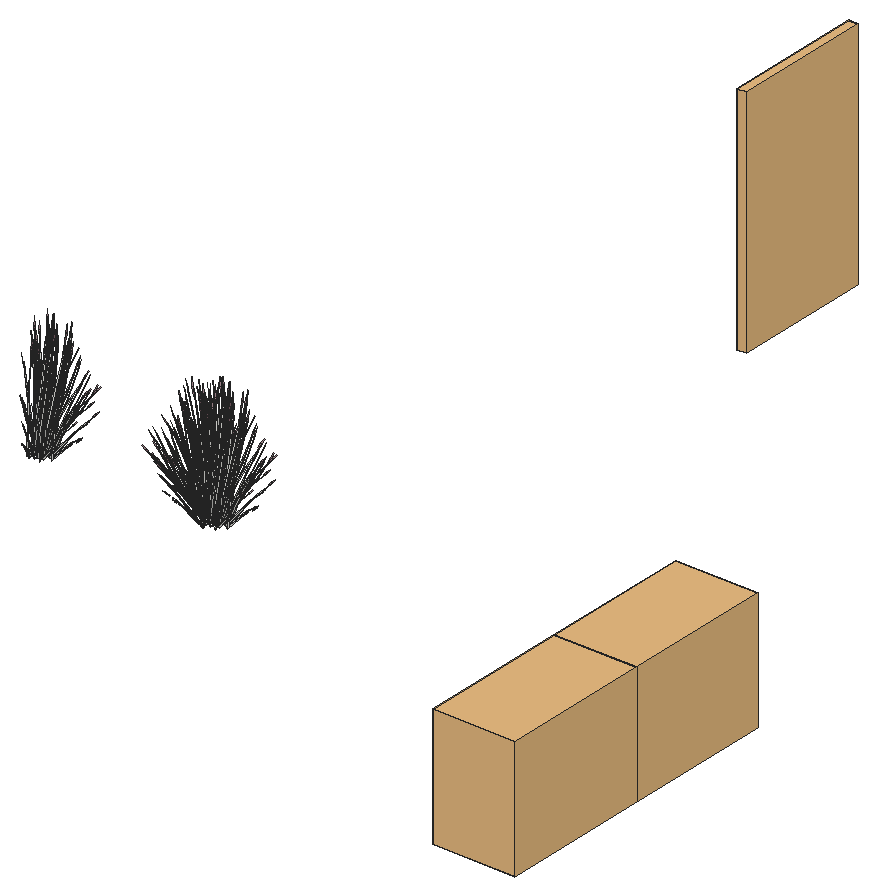
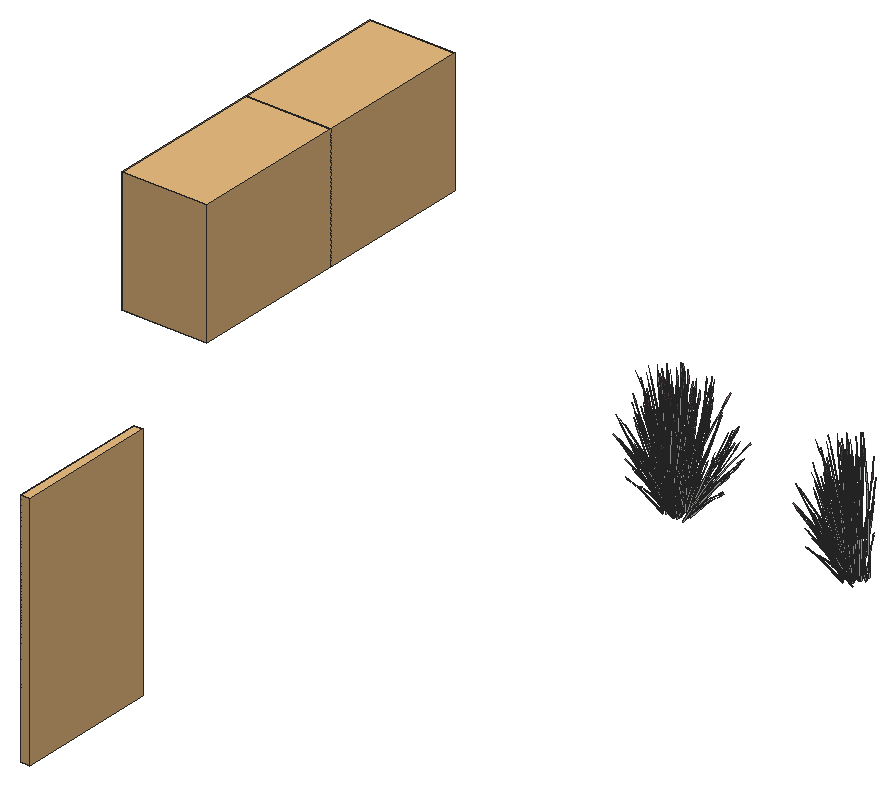
# SketchUp Ruby script. Lengths in millimetres.
U = 1.mm
M = Sketchup.active_model
def pt(a) = Geom::Point3d.new(a.map { |v| v * U })
def face(e, loops, mat)
  f = e.add_face(loops[0].map { |a| pt(a) })
  loops[1..].each { |l| e.add_face(l.map { |a| pt(a) }).erase! }
  f.material = f.back_material = mat if mat
  f
end
# faces: each face lists its corners as indices into pts; further lists are holes
def faces(e, pts, list, mat = nil) = list.each { |f| face(e, (f[0].is_a?(Array) ? f : [f]).map { |l| l.map { |i| pts[i] } }, mat) }
# xy, xz, yz: faces in a plane at the given z, y or x. An outline is a flat list of corners, or four numbers for a rectangle; further outlines are holes
def ring(l) = l.size == 4 ? [[l[0], l[1]], [l[2], l[1]], [l[2], l[3]], [l[0], l[3]]] : l.each_slice(2).to_a
def flat(e, list, mat, &to3) = list.each { |f| face(e, (f[0].is_a?(Array) ? f : [f]).map { |l| ring(l).map { |u, v| to3.(u, v) } }, mat) }
def xy(e, z, list, mat = nil) = flat(e, list, mat) { |x, y| [x, y, z] }
def xz(e, y, list, mat = nil) = flat(e, list, mat) { |x, z| [x, y, z] }
def yz(e, x, list, mat = nil) = flat(e, list, mat) { |y, z| [x, y, z] }
def lines(e, pts, list) = list.each { |a, b| e.add_line(pt(pts[a]), pt(pts[b])) }
# prism: a flat outline (further loops are holes) pulled along v
def prism(e, loops, v, mat = nil)
  f = face(e, loops, mat); d = Geom::Vector3d.new(v.map { |x| x * U })
  f.pushpull(f.normal.samedirection?(d) ? d.length : -d.length)
end
def box(e, o, s, mat = nil) = prism(e, [[o, [o[0] + s[0], o[1], o[2]], [o[0] + s[0], o[1] + s[1], o[2]], [o[0], o[1] + s[1], o[2]]]], [0, 0, s[2]], mat)
def at(x, y, z, deg = 0) = Geom::Transformation.translation(pt([x, y, z])) * Geom::Transformation.rotation(ORIGIN, Z_AXIS, deg.degrees)
def axes(o, x, y, z) = Geom::Transformation.new([*x, 0, *y, 0, *z, 0, *pt(o).to_a, 1])
def part(name) = M.definitions.add(name)
# library, detail: a bought-in or finely detailed component or shape, given as its bounding box
def library(name, o, s) = part(name).tap { |d| box(d.entities, o, s) }
def detail(e, o, s) = box(e.add_group.entities, o, s)
def put(e, d, t, mat = nil) = e.add_instance(d, t).tap { |i| i.material = mat if mat }
def group(e, t, mat = nil) = e.add_group.tap { |g| g.transformation = t; g.material = mat if mat }.entities
root = M.entities
M.materials.add("LightPink_Translucent").color = [144, 107, 117]
M.materials["LightPink_Translucent"].alpha = 0.8
c1 = part("blade")
p = [[54.7,5.3,558.8],[0,4.4,0],[2.3,11.5,0],[55.5,7.8,558.8],[58.2,7.8,558.8],[9.8,11.5,0],
  [62.9,5.7,838.2],[63,6,838.2],[63.4,6,838.2]]
faces(c1.entities,p,[[0,1,2,3],[4,5,2,3],[6,0,3,7],[7,3,4,8]])
c2 = part("seeds")
p = [[7.6,-2.7,35.1],[-0.2,-0.6,40.4],[-0.2,-0.8,0.9],[3.5,-1.8,-1.7],[7.5,-0.8,76.3],[3.7,0.2,78.9]]
faces(c2.entities,p,[[0,1,2,3],[1,0,4,5]],"LightPink_Translucent")
c3 = part("blade with seeds")
put(c3.entities,c1,at(0,0,0))
put(c3.entities,c2,axes([60.9,6.5,787.2],[1.5799,-0.05474,1.17369],[-0.12525,1.92788,0.29478],[-0.07173,-0.02425,1.56792]))
c4 = library("porta+4",[5.1,-137.5,33.9],[1182.3,119.8,2113.3])
c5 = library("Ornamental gate leaf",[0,0,0],[4100,1077.8,7119.6])
c6 = part("cong")
put(c6.entities,c5,axes([6217.3,5957.9,0],[-1,0,0],[0,1,0],[0,0,1]))
put(c6.entities,c5,at(6217.3,5957.9,0))
put(root,c3,axes([10117.4,4303.7,60],[0.53281,1.15808,0.45755],[-1.52239,0.4027,0.17955],[0.01861,-0.2128,1.58856]))
put(root,c3,axes([10111.2,4299.9,56.2],[0.59459,-0.93321,-0.44739],[1.23546,0.44912,0.21531],[0,-0.21512,1.43643]))
put(root,c3,axes([10149.9,4376.4,56],[-0.39985,-0.89288,0],[1.1418,-0.31268,0],[0,0,1.54371]))
put(root,c3,axes([10113,4424.2,37.9],[0.19833,-0.05635,1.76342],[1.19302,0.31018,-0.26939],[0.03489,0.3496,0.30037]))
put(root,c3,axes([10119.7,4432.2,115],[-0.36946,0.79643,-0.35414],[-1.07787,-0.23229,0.4572],[0.09883,0.32066,0.87481]))
put(root,c3,axes([10190.9,4331.6,56.2],[-0.59459,0.93321,-0.44739],[-1.23546,-0.44912,0.21531],[0,0.21512,1.43643]))
put(root,c3,axes([10250.6,4317.2,62.8],[-0.96285,-0.75439,0.17642],[0.97031,-0.7317,0.35086],[-0.10634,0.15406,1.60407]))
put(root,c3,axes([10166.1,4306.1,56],[0,-1.19833,0],[1.53239,0,0],[0,0,1.79456]))
put(root,c3,axes([10129.9,4311.7,61.8],[1.3808,0.50196,0.24065],[-0.66454,1.04299,0.50002],[0,-0.24043,1.60543]))
put(root,c3,axes([10185.7,4318.3,58.2],[0,1.19774,-0.05637],[-1.53239,0,0],[0,0.03764,1.79368]))
put(root,c3,axes([10118.6,4293.9,69],[-1.33077,0.06393,0.44739],[-0.12035,-1.06125,-0.21531],[0.23824,-0.10756,1.43643]))
put(root,c3,axes([10102.8,4247.7,62.8],[-0.35402,1.02926,0.17642],[-1.29548,-0.29127,0.35086],[0.22379,-0.00501,1.60407]))
put(root,c3,axes([10167.1,4377.2,58.2],[0.53281,1.18979,-0.06012],[-1.52239,0.41691,0],[0.01861,0.04155,1.72173]))
put(root,c3,axes([10086.7,4215.4,60.3],[-0.7662,-1.03778,0],[1.28187,-0.57875,-0.51607],[0.29196,-0.13181,1.63711]))
put(root,c3,axes([10122.5,4414.1,126.5],[0.5849,0.8421,-0.71045],[-1.20401,0.4693,0.08574],[0.13677,0.40688,1.00501]))
put(root,c3,axes([10278.8,4337.5,55.9],[-1.53164,-0.00828,-0.04976],[0,-1.1575,0.49943],[-0.04813,0.2635,1.58352]))
put(root,c3,axes([10202.4,4249.1,62.8],[-1.31687,0.27488,0.17642],[-0.32517,-1.02297,0.35086],[0.11745,0.14905,1.60407]))
put(root,c3,axes([10168.2,4151.7,70.2],[0.15721,0.60392,1.1486],[-0.87211,-0.33448,0.84392],[0.09385,-0.30923,0.25299]))
put(root,c3,axes([10147.7,4287,60],[-1.01611,0.93987,0.45755],[-1.20717,-0.82966,0.17955],[0.24496,-0.0938,1.58856]))
put(root,c3,axes([10191.7,4324.6,56.2],[0.85545,0.66896,0],[-0.85545,0.66896,0],[0,0,1.69266]))
put(root,c3,axes([10191.4,4304.7,69],[0.59459,-0.93321,0.44739],[1.23546,0.44912,-0.21531],[0,0.21512,1.43643]))
put(root,c3,axes([10178.3,4387.1,56],[1.23546,0.46496,0],[-0.59459,0.96613,0],[0,0,1.74954]))
put(root,c3,axes([10133.6,4418.4,118.9],[1.20468,0.25962,-0.51099],[-0.41292,0.89013,-0.3958],[0.11046,0.35838,0.97773]))
put(root,c3,axes([10181.3,4299.1,60.5],[-1.54892,-0.2182,0.49198],[0.31522,-1.23236,0.19306],[0.22636,0.119,1.70813]))
put(root,c3,axes([10270.7,4341.8,51.5],[-0.85545,0.64616,-0.30978],[-0.85545,-0.64616,0.30978],[0,0.20813,1.38974]))
put(root,c3,axes([10208.6,4338.8,53.2],[0.44936,0.94823,-0.69212],[-1.29441,0.3415,-0.18165],[0.04967,0.32109,1.52773]))
put(root,c3,axes([10192.5,4313,56],[1.37109,0,0],[0,1.07219,0],[0,0,1.78407]))
put(root,c3,axes([10159,4282.9,69],[-0.73619,-0.86927,0.44739],[1.11511,-0.61213,-0.21531],[0.23824,0.10756,1.43643]))
put(root,c3,axes([10125,4288.2,67.7],[-0.1428,-1.18174,-0.29095],[1.48733,-0.07145,-0.50002],[0.26191,-0.15741,1.59708]))
put(root,c3,axes([10204.6,4310.2,66.5],[1.1418,-0.30203,0.1448],[0.39985,0.86246,-0.41347],[0,0.18981,1.26744]))
put(root,c3,axes([10215.4,4225.5,118.9],[-0.87728,-0.69587,-0.51099],[0.92674,-0.60943,-0.3958],[0.13348,-0.35356,0.97773]))
put(root,c3,axes([10194.6,4311.9,67.7],[1.38012,0.49416,-0.29095],[-0.66454,1.04299,-0.50002],[0.04337,0.25608,1.59708]))
put(root,c3,axes([10120,4221.7,51.5],[1.14332,0.25625,-0.30978],[-0.28787,0.90242,0.30978],[0.23049,-0.10406,1.38974]))
put(root,c3,axes([10200.8,4194.1,65.8],[-0.34835,0.20963,1.43002],[-1.04325,-0.36691,-0.30754],[0.19338,-0.4563,0.61141]))
put(root,c3,axes([10270.7,4318,63],[0,-1.03566,0.49651],[1.37109,0,0],[0,0.23588,1.57504]))
put(root,c3,axes([10285.7,4342.4,51.2],[0,1.03566,-0.49651],[-1.37109,0,0],[0,0.23588,1.57504]))
put(root,c3,axes([10113.2,4211.3,51.2],[1.14694,-0.51783,-0.49651],[0.68554,0.92854,0],[0.26122,-0.11794,1.57504]))
put(root,c3,axes([10151,4371.7,98.5],[-0.28013,-0.33252,1.71376],[1.29445,-0.27994,0.13857],[0.29256,0.52202,0.73262]))
put(root,c3,axes([10171.6,4276.7,66.5],[0.23642,-0.92427,0.1448],[1.15506,0.16044,-0.41347],[0.21021,0.09491,1.26744]))
put(root,c3,axes([10213.3,4235.8,63],[-1.14694,-0.51783,0.49651],[0.68554,-0.92854,0],[0.26122,0.11794,1.57504]))
put(root,c3,axes([10222.3,4233.5,126.5],[0.03189,-0.95798,-0.71045],[1.34277,0.06434,0.08574],[0.14171,-0.40585,1.00501]))
put(root,c3,axes([10187.9,4373.2,55.5],[1.2866,-0.3514,-0.19198],[0.45209,1.01223,0.00008],[0.14202,-0.03884,1.73897]))
put(root,c3,axes([10188.5,4296.7,56.2],[0.73619,0.86927,-0.44739],[-1.11511,0.61213,0.21531],[0.23824,0.10756,1.43643]))
put(root,c3,axes([10236.4,4218.9,115],[0.82919,-0.54528,-0.35414],[0.78493,0.62262,0.4572],[0.11943,-0.31634,0.87481]))
put(root,c3,axes([10241.4,4397,70.2],[-0.69001,-0.29779,1.1486],[0.89096,-0.30257,0.84392],[0.24031,0.2563,0.25299]))
put(root,c3,axes([10179,4388.9,65.8],[0.02163,-0.34331,1.43002],[1.03345,-0.38348,-0.30754],[0.31903,0.4109,0.61141]))
put(root,c3,axes([10147.7,4265.3,52.3],[0.82544,-0.77843,-0.62353],[1.0254,0.70586,-0.16365],[0.33076,-0.19418,1.37633]))
put(root,c3,axes([10239.7,4247.7,51.5],[0.28787,0.90242,-0.30978],[-1.14332,0.25625,0.30978],[0.23049,0.10406,1.38974]))
put(root,c3,axes([10294.4,4322.4,60.4],[1.53239,0,0],[0,1.1575,-0.51607],[0,0.26363,1.63711]))
put(root,c3,axes([10168.6,4284.3,67.7],[1.23732,-0.68758,-0.29095],[0.8228,0.97154,-0.50002],[0.30528,0.09867,1.59708]))
put(root,c3,axes([10244.2,4431.4,67.7],[-0.78586,-0.03248,1.0506],[0.51898,-0.68985,0.58006],[0.31045,0.24509,0.8241]))
put(root,c3,axes([10184,4221.2,98.5],[-0.22818,0.35597,1.71376],[-0.95725,-0.73667,0.13857],[0.43183,-0.45914,0.73262]))
put(root,c3,axes([10089.2,4268.8,40.5],[-1.20625,0.41464,1.28929],[-0.38394,-1.1897,0.50096],[0.74071,0.01979,1.46642]))
put(root,c3,axes([10201.8,4407.4,118.9],[1.20928,-0.24619,-0.51099],[0.21154,0.93233,-0.3958],[0.32481,0.26718,0.97773]))
put(root,c3,axes([10230.1,4222,60.4],[0.7662,-1.03778,0],[1.28187,0.57875,-0.51607],[0.29196,0.13181,1.63711]))
put(root,c3,axes([10262.7,4210.5,37.9],[-0.18342,-0.08159,1.76342],[-0.47115,-0.9115,-0.26939],[0.31784,-0.24736,0.30037]))
put(root,c3,axes([10247.8,4237.9,51.2],[1.14694,0.51783,-0.49651],[-0.68554,0.92854,0],[0.26122,0.11794,1.57504]))
put(root,c3,axes([10246.4,4425,37.9],[0.08928,-0.14952,1.76342],[1.12407,-0.44035,-0.26939],[0.34078,0.22791,0.30037]))
put(root,c3,axes([10261.7,4266.1,118.9],[-0.31482,-0.94565,-0.51099],[1.19224,-0.16542,-0.3958],[0.34166,-0.254,0.97773]))
put(root,c3,axes([10315,4390.1,99.8],[-0.23455,-0.87059,-0.03492],[1.10861,-0.20015,-0.15832],[0.23151,0.05519,0.52218]))
put(root,c3,axes([10205.3,4288.3,52.3],[1.27479,0.1698,-0.62353],[-0.26901,1.04736,-0.16365],[0.38043,0.12691,1.37633]))
put(root,c3,axes([10343.2,4304,57.4],[-0.75977,-0.66224,-0.06488],[0.83212,-0.6068,-0.29416],[0.23578,-0.04272,0.97024]))
put(root,c3,axes([10298.9,4218.4,70.2],[-0.40819,0.5272,1.1486],[-0.35086,-0.70831,0.84392],[0.33713,-0.17749,0.25299]))
put(root,c3,axes([10198.6,4345.3,98.5],[-0.45521,-0.17844,1.71376],[0.94204,-0.74856,0.13857],[0.58713,0.33769,0.73262]))
put(root,c3,axes([10284,4268.7,115],[1.06674,-0.14801,-0.35414],[0.28168,0.84611,0.4572],[0.30569,-0.22726,0.87481]))
put(root,c3,axes([10262.5,4275.8,126.5],[0.64013,-0.81717,-0.71045],[1.12174,0.58074,0.08574],[0.38221,-0.29607,1.00501]))
put(root,c3,axes([10262.2,4387.6,115],[0.69728,0.64842,-0.35414],[-0.79619,0.61382,0.4572],[0.40453,0.09339,0.87481]))
put(root,c3,axes([10275.8,4319.5,118.9],[0.332,-0.94205,-0.51099],[1.13828,0.3229,-0.3958],[0.45829,-0.08638,0.97773]))
put(root,c3,axes([10348.4,4334.7,70.2],[-0.75718,0.17097,1.1486],[0.35641,-0.70661,0.84392],[0.40168,0.04835,0.25299]))
put(root,c3,axes([10286.1,4256.8,65.8],[-0.4378,-0.03068,1.43002],[-0.44851,-0.8229,-0.30754],[0.53783,-0.23279,0.61141]))
put(root,c3,axes([10293.5,4330.4,115],[1.01846,0.28891,-0.35414],[-0.29705,0.84289,0.4572],[0.41005,-0.07729,0.87481]))
put(root,c3,axes([10243.5,4376.6,126.5],[1.22504,0.02494,-0.71045],[-0.08228,1.05005,0.08574],[0.51899,0.11081,1.00501]))
put(root,c3,axes([10306.7,4326.2,50.4],[-0.7893,0.12429,1.41583],[-0.12563,-0.9893,0.08104],[0.55282,-0.14974,0.80566]))
put(root,c3,axes([10328.5,4309.8,37.9],[-0.06405,-0.15723,1.76342],[0.44421,-0.91974,-0.26939],[0.4481,-0.01323,0.30037]))
put(root,c3,axes([10223,4303.9,98.5],[-0.50831,0.02346,1.71376],[0.33721,-1.01661,0.13857],[0.72439,0.06288,0.73262]))
put(root,c3,axes([10270.3,4328.2,126.5],[1.07686,-0.45739,-0.71045],[0.60013,0.94154,0.08574],[0.52031,-0.10696,1.00501]))
put(root,c3,axes([10312.3,4363.5,65.8],[-0.29514,-0.25472,1.43002],[0.38401,-0.84262,-0.30754],[0.59714,0.11414,0.61141]))
put(root,c3,axes([12280.5,4290.3,98.5],[0.50831,-0.02346,1.71376],[-0.33721,1.01661,0.13857],[-0.72439,-0.06288,0.73262]))
put(root,c3,axes([12285.9,4335.8,98.5],[0.42521,-0.21906,1.71376],[0.35798,1.01226,0.13857],[-0.66754,0.22878,0.73262]))
put(root,c3,axes([12252.2,4379.6,65.8],[0.42589,0.08502,1.43002],[0.2745,0.86839,-0.30754],[-0.57851,0.16255,0.61141]))
put(root,c3,axes([12347.9,4308.9,84.9],[0.34834,-0.14982,1.77064],[0.12012,1.04605,0.13857],[-0.75452,0.1388,0.63284]))
put(root,c3,axes([12319.1,4266.3,126.5],[-1.22504,-0.02494,-0.71045],[0.08228,-1.05005,0.08574],[-0.51899,-0.11081,1.00501]))
put(root,c3,axes([12294,4272.8,65.8],[0.23927,0.28834,1.43002],[-0.55135,0.78376,-0.30754],[-0.56612,-0.18733,0.61141]))
put(root,c3,axes([12269.1,4312.5,115],[-1.01846,-0.28891,-0.35414],[0.29705,-0.84289,0.4572],[-0.41005,0.07729,0.87481]))
put(root,c3,axes([12304.9,4248.9,98.5],[0.45521,0.17844,1.71376],[-0.94204,0.74856,0.13857],[-0.58713,-0.33769,0.73262]))
put(root,c3,axes([12286.9,4323.4,118.9],[-0.332,0.94205,-0.51099],[-1.13828,-0.3229,-0.3958],[-0.45829,0.08638,0.97773]))
put(root,c3,axes([12308.8,4271.7,118.9],[-0.88986,0.68603,-0.51099],[-0.77932,-0.72471,-0.3958],[-0.45212,-0.10438,0.97773]))
put(root,c3,axes([12272.3,4321.9,37.9],[0.03108,0.16322,1.76342],[-0.62654,0.85237,-0.26939],[-0.44504,-0.04296,0.30037]))
put(root,c3,axes([12229.7,4425.8,70.2],[0.51072,-0.46938,1.1486],[0.20153,0.74307,0.84392],[-0.36908,0.13305,0.25299]))
put(root,c3,axes([12300.4,4255.4,115],[-0.69728,-0.64842,-0.35414],[0.79619,-0.61382,0.4572],[-0.40453,-0.09339,0.87481]))
put(root,c3,axes([12325.4,4353.1,98.5],[0.30609,-0.31822,1.71376],[0.77286,0.85893,0.13857],[-0.53009,0.39116,0.73262]))
put(root,c3,axes([12278.6,4374.2,115],[-1.06674,0.14801,-0.35414],[-0.28168,-0.84611,0.4572],[-0.30569,0.22726,0.87481]))
put(root,c3,axes([12263.8,4438,37.9],[0.16438,0.10347,1.76342],[0.27873,0.95868,-0.26939],[-0.36432,0.20444,0.30037]))
put(root,c3,axes([12257.9,4294.8,70.2],[0.78239,-0.07411,1.1486],[-0.49629,0.65296,0.84392],[-0.38663,-0.09795,0.25299]))
put(root,c3,axes([12319.6,4373,98.5],[0.22818,-0.35597,1.71376],[0.95725,0.73667,0.13857],[-0.43183,0.45914,0.73262]))
put(root,c3,axes([12300.9,4376.8,118.9],[0.31482,0.94565,-0.51099],[-1.19224,0.16542,-0.3958],[-0.34166,0.254,0.97773]))
put(root,c3,axes([12376.4,4359.5,52.3],[-1.27479,-0.1698,-0.62353],[0.26901,-1.04736,-0.16365],[-0.38043,-0.12691,1.37633]))
put(root,c3,axes([12373.2,4234.9,126.5],[-1.04497,-0.50058,-0.71045],[0.74264,-0.8772,0.08574],[-0.3786,-0.29889,1.00501]))
put(root,c3,axes([12360.8,4235.5,118.9],[-1.20928,0.24619,-0.51099],[-0.21154,-0.93233,-0.3958],[-0.32481,-0.26718,0.97773]))
put(root,c3,axes([12334,4409.9,51.2],[-1.14694,-0.51783,-0.49651],[0.68554,-0.92854,0],[-0.26122,-0.11794,1.57504]))
put(root,c3,axes([12321.2,4214,37.9],[-0.11871,0.13643,1.76342],[-1.19964,0.29415,-0.26939],[-0.2898,-0.26759,0.30037]))
put(root,c3,axes([12351.7,4425.8,60.3],[-0.7662,1.03778,0],[-1.28187,-0.57875,-0.51607],[-0.29196,-0.13181,1.63711]))
put(root,c3,axes([12316.2,4463.9,65.8],[0.38672,-0.16338,1.43002],[0.95481,0.49262,-0.30754],[-0.28419,0.42626,0.61141]))
put(root,c3,axes([12302.2,4227.3,54.1],[-0.35352,0.84566,-0.03893],[-1.08806,-0.26014,-0.17649],[-0.1652,-0.13832,0.58215]))
put(root,c3,axes([12343.5,4200.2,65.8],[-0.07421,0.33879,1.43002],[-1.08488,0.28361,-0.30754],[-0.25359,-0.4379,0.61141]))
put(root,c3,axes([12352.5,4222.5,98.5],[0.28013,0.33252,1.71376],[-1.29445,0.27994,0.13857],[-0.29256,-0.52202,0.73262]))
put(root,c3,axes([12413.2,4363.5,67.7],[-1.23732,0.68758,-0.29095],[-0.8228,-0.97154,-0.50002],[-0.30528,-0.09867,1.59708]))
put(root,c3,axes([12364,4218.1,115],[-0.18927,-0.83419,-0.35414],[1.08199,-0.22027,0.4572],[-0.29062,-0.23905,0.87481]))
put(root,c3,axes([12287.4,4325.4,60.3],[-1.53239,0,0],[0,-1.1575,-0.51607],[0,-0.26363,1.63711]))
put(root,c3,axes([12342.1,4400.1,51.5],[-0.28787,-0.90242,-0.30978],[1.14332,-0.25625,0.30978],[-0.23049,-0.10406,1.38974]))
put(root,c3,axes([12326.3,4424,115],[-0.82919,0.54528,-0.35414],[-0.78493,-0.62262,0.4572],[-0.11943,0.31634,0.87481]))
put(root,c3,axes([12434,4382.5,52.3],[-0.82544,0.77843,-0.62353],[-1.0254,-0.70586,-0.16365],[-0.33076,0.19418,1.37633]))
put(root,c3,axes([12317.5,4317.6,59.2],[-1.1399,0.87071,0.30756],[-1.1406,-0.86155,-0.36492],[-0.03981,-0.24727,1.64885]))
put(root,c3,axes([12436.7,4378.8,84.5],[1.05902,0.41762,1.51261],[-1.03748,0.89969,0.59816],[-0.46471,-0.53324,1.26806]))
put(root,c3,axes([12334,4186.4,70.2],[0.63926,0.36046,1.1486],[-0.93099,0.21668,0.84392],[-0.1992,-0.27702,0.25299]))
put(root,c3,axes([12448.5,4371.4,62.6],[-1.19666,-0.83357,-0.25192],[1.00694,-0.93603,0.5513],[-0.32224,0.09751,1.68216]))
put(root,c3,axes([12393.2,4351.1,56.2],[-0.73619,-0.86927,-0.44739],[1.11511,-0.61213,0.21531],[-0.23824,-0.10756,1.43643]))
put(root,c3,axes([12340.3,4409.4,135.6],[-0.03189,0.95798,-0.7886],[-1.34277,-0.06434,0.09517],[-0.14171,0.40585,1.11556]))
put(root,c3,axes([12339.7,4477.8,70.2],[-0.03171,-0.6158,1.1486],[0.7925,0.43922,0.84392],[-0.15586,0.29352,0.25299]))
put(root,c3,axes([12433.1,4366.9,56.2],[-1.33077,0.06393,-0.44739],[-0.12035,-1.06125,0.21531],[-0.23824,0.10756,1.43643]))
put(root,c3,axes([12368.5,4412,63],[1.14694,0.51783,0.49651],[-0.68554,0.92854,0],[-0.26122,-0.11794,1.57504]))
put(root,c3,axes([12328.9,4443.6,85.4],[0.02693,-0.53464,1.54345],[1.21102,0.2824,0.21329],[-0.10493,0.5698,0.72882]))
put(root,c3,axes([12396,4363.7,61.9],[0.32481,-1.2272,-0.23429],[1.54007,0.21392,0.51271],[-0.26911,-0.16947,1.5644]))
put(root,c3,axes([12410.2,4371.1,66.5],[-0.23642,0.92427,0.1448],[-1.15506,-0.16044,-0.41347],[-0.21021,-0.09491,1.26744]))
put(root,c3,axes([12468.6,4436.5,51.2],[-1.14694,0.51783,-0.49651],[-0.68554,-0.92854,0],[-0.26122,0.11794,1.57504]))
put(root,c3,axes([12296.1,4305.4,51.2],[0,-1.03566,-0.49651],[1.37109,0,0],[0,-0.23588,1.57504]))
put(root,c3,axes([12311,4329.8,63],[0,1.03566,0.49651],[-1.37109,0,0],[0,-0.23588,1.57504]))
put(root,c3,axes([12470.5,4429.4,55.7],[-0.75665,-1.04141,-0.05142],[1.28187,-0.57875,0.51607],[-0.31588,0.09915,1.6363]))
put(root,c3,axes([12347.2,4417.5,127.1],[0.87728,0.69587,-0.5672],[-0.92674,0.60943,-0.43934],[-0.13348,0.35356,1.08528]))
put(root,c3,axes([12461.8,4426.1,51.5],[-1.14332,-0.25625,-0.30978],[0.28787,-0.90242,0.30978],[-0.23049,0.10406,1.38974]))
put(root,c3,axes([12387.1,4335.9,67.7],[-1.38012,-0.49416,-0.29095],[0.66454,-1.04299,-0.50002],[-0.04337,-0.25608,1.59708]))
put(root,c3,axes([12478.4,4328.1,72.2],[-0.03348,-0.97511,1.41272],[1.51511,0.25277,0.59816],[-0.35835,0.53357,1.3335]))
put(root,c3,axes([12323,4444,71.7],[1.11329,-0.1834,0.06507],[0.25594,0.73887,-0.86304],[-0.07058,0.37403,0.7736]))
put(root,c3,axes([12456.8,4359.6,67.7],[0.1428,1.18174,-0.29095],[-1.48733,0.07145,-0.50002],[-0.26191,0.15741,1.59708]))
put(root,c3,axes([12371.5,4309.2,53.3],[-0.50328,-1.06202,-0.69835],[1.44974,-0.38248,-0.18329],[-0.05563,-0.35963,1.54149]))
put(root,c3,axes([12429,4224.5,118.9],[-1.20468,-0.25962,-0.51099],[0.41292,-0.89013,-0.3958],[-0.11046,-0.35838,0.97773]))
put(root,c3,axes([12372.6,4392.1,98.5],[-0.02999,-0.3975,1.71376],[1.30002,0.26369,0.13857],[-0.08041,0.56647,0.73262]))
put(root,c3,axes([12311,4306,51.5],[0.85545,-0.64616,-0.30978],[0.85545,0.64616,0.30978],[0,-0.20813,1.38974]))
put(root,c3,axes([12409.2,4199.9,54.1],[-0.84686,0.59414,-0.03893],[-0.77596,-0.65071,-0.17649],[-0.05463,-0.18438,0.58215]))
put(root,c3,axes([12400.5,4348.7,60],[1.54892,0.2182,0.45755],[-0.31522,1.23236,0.17955],[-0.22636,-0.119,1.58856]))
put(root,c3,axes([12390.3,4343.1,69],[-0.59459,0.93321,0.44739],[-1.23546,-0.44912,-0.21531],[0,-0.21512,1.43643]))
put(root,c3,axes([12440.2,4228.8,126.5],[-0.5849,-0.8421,-0.71045],[1.20401,-0.4693,0.08574],[-0.13677,-0.40688,1.00501]))
put(root,c3,axes([12379.4,4398.7,62.8],[1.31687,-0.27488,0.17642],[0.32517,1.02297,0.35086],[-0.11745,-0.14905,1.60407]))
put(root,c3,axes([12422.4,4402.9,55.8],[-1.23546,-0.46496,0],[0.59459,-0.96613,0],[0,0,1.62707]))
put(root,c3,axes([12495,4432.4,60.3],[0.7662,1.03778,0],[-1.28187,0.57875,-0.51607],[-0.29196,0.13181,1.63711]))
put(root,c3,axes([12478.9,4400.1,62.8],[0.35402,-1.02926,0.17642],[1.29548,0.29127,0.35086],[-0.22379,0.00501,1.60407]))
put(root,c3,axes([12463.7,4365.5,66.5],[0.90538,0.62224,0.1448],[-0.75521,0.70202,-0.41347],[-0.21021,0.09491,1.26744]))
put(root,c3,axes([12455.5,4346,58.4],[-1.1399,-0.8914,-0.06131],[1.1406,-0.89194,0],[-0.03981,-0.03113,1.75571]))
put(root,c3,axes([12463.2,4353.9,69],[1.33077,-0.06393,0.44739],[0.12035,1.06125,-0.21531],[-0.23824,0.10756,1.43643]))
put(root,c3,axes([12471.4,4415.9,59.2],[1.53422,0.33662,0.30756],[-0.38383,1.20322,-0.36492],[-0.25393,0.15059,1.64885]))
put(root,c3,axes([12414.5,4181.4,37.9],[-0.20555,0.03731,1.76342],[-1.13672,-0.42002,-0.26939],[0.01907,-0.35034,0.30037]))
put(root,c3,axes([12488.2,4414.2,63],[1.14694,-0.51783,0.49651],[0.68554,0.92854,0],[-0.26122,0.11794,1.57504]))
put(root,c3,axes([12443,4210.7,115],[0.36946,-0.79643,-0.35414],[1.07787,0.23229,0.4572],[-0.09883,-0.32066,0.87481]))
put(root,c3,axes([12397.1,4319.9,60],[0.53281,1.15808,0.45755],[-1.52239,0.4027,0.17955],[0.01861,-0.2128,1.58856]))
put(root,c3,axes([12390.9,4316.2,56.2],[0.59459,-0.93321,-0.44739],[1.23546,0.44912,0.21531],[0,-0.21512,1.43643]))
put(root,c3,axes([12429.6,4392.6,56],[-0.39985,-0.89288,0],[1.1418,-0.31268,0],[0,0,1.54371]))
put(root,c3,axes([12392.7,4440.4,37.9],[0.19833,-0.05635,1.76342],[1.19302,0.31018,-0.26939],[0.03489,0.3496,0.30037]))
put(root,c3,axes([12399.4,4448.5,115],[-0.36946,0.79643,-0.35414],[-1.07787,-0.23229,0.4572],[0.09883,0.32066,0.87481]))
put(root,c3,axes([12470.6,4347.9,56.2],[-0.59459,0.93321,-0.44739],[-1.23546,-0.44912,0.21531],[0,0.21512,1.43643]))
put(root,c3,axes([12530.3,4333.4,62.8],[-0.96285,-0.75439,0.17642],[0.97031,-0.7317,0.35086],[-0.10634,0.15406,1.60407]))
put(root,c3,axes([12445.8,4322.4,56],[0,-1.19833,0],[1.53239,0,0],[0,0,1.79456]))
put(root,c3,axes([12409.6,4327.9,61.8],[1.3808,0.50196,0.24065],[-0.66454,1.04299,0.50002],[0,-0.24043,1.60543]))
put(root,c3,axes([12465.3,4334.5,58.2],[0,1.19774,-0.05637],[-1.53239,0,0],[0,0.03764,1.79368]))
put(root,c3,axes([12398.3,4310.2,69],[-1.33077,0.06393,0.44739],[-0.12035,-1.06125,-0.21531],[0.23824,-0.10756,1.43643]))
put(root,c3,axes([12382.5,4263.9,62.8],[-0.35402,1.02926,0.17642],[-1.29548,-0.29127,0.35086],[0.22379,-0.00501,1.60407]))
put(root,c3,axes([12446.7,4393.4,58.2],[0.53281,1.18979,-0.06012],[-1.52239,0.41691,0],[0.01861,0.04155,1.72173]))
put(root,c3,axes([12366.4,4231.6,60.3],[-0.7662,-1.03778,0],[1.28187,-0.57875,-0.51607],[0.29196,-0.13181,1.63711]))
put(root,c3,axes([12402.2,4430.3,126.5],[0.5849,0.8421,-0.71045],[-1.20401,0.4693,0.08574],[0.13677,0.40688,1.00501]))
put(root,c3,axes([12558.5,4353.8,55.9],[-1.53164,-0.00828,-0.04976],[0,-1.1575,0.49943],[-0.04813,0.2635,1.58352]))
put(root,c3,axes([12482.1,4265.3,62.8],[-1.31687,0.27488,0.17642],[-0.32517,-1.02297,0.35086],[0.11745,0.14905,1.60407]))
put(root,c3,axes([12447.9,4167.9,70.2],[0.15721,0.60392,1.1486],[-0.87211,-0.33448,0.84392],[0.09385,-0.30923,0.25299]))
put(root,c3,axes([12427.3,4303.2,60],[-1.01611,0.93987,0.45755],[-1.20717,-0.82966,0.17955],[0.24496,-0.0938,1.58856]))
put(root,c3,axes([12471.4,4340.9,56.2],[0.85545,0.66896,0],[-0.85545,0.66896,0],[0,0,1.69266]))
put(root,c3,axes([12471.1,4321,69],[0.59459,-0.93321,0.44739],[1.23546,0.44912,-0.21531],[0,0.21512,1.43643]))
put(root,c3,axes([12458,4403.3,56],[1.23546,0.46496,0],[-0.59459,0.96613,0],[0,0,1.74954]))
put(root,c3,axes([12413.3,4434.6,118.9],[1.20468,0.25962,-0.51099],[-0.41292,0.89013,-0.3958],[0.11046,0.35838,0.97773]))
put(root,c3,axes([12460.9,4315.3,60.5],[-1.54892,-0.2182,0.49198],[0.31522,-1.23236,0.19306],[0.22636,0.119,1.70813]))
put(root,c3,axes([12550.4,4358,51.5],[-0.85545,0.64616,-0.30978],[-0.85545,-0.64616,0.30978],[0,0.20813,1.38974]))
put(root,c3,axes([12488.3,4355,53.2],[0.44936,0.94823,-0.69212],[-1.29441,0.3415,-0.18165],[0.04967,0.32109,1.52773]))
put(root,c3,axes([12472.2,4329.2,56],[1.37109,0,0],[0,1.07219,0],[0,0,1.78407]))
put(root,c3,axes([12438.7,4299.1,69],[-0.73619,-0.86927,0.44739],[1.11511,-0.61213,-0.21531],[0.23824,0.10756,1.43643]))
put(root,c3,axes([12404.7,4304.4,67.7],[-0.1428,-1.18174,-0.29095],[1.48733,-0.07145,-0.50002],[0.26191,-0.15741,1.59708]))
put(root,c3,axes([12484.2,4326.4,66.5],[1.1418,-0.30203,0.1448],[0.39985,0.86246,-0.41347],[0,0.18981,1.26744]))
put(root,c3,axes([12495.1,4241.7,118.9],[-0.87728,-0.69587,-0.51099],[0.92674,-0.60943,-0.3958],[0.13348,-0.35356,0.97773]))
put(root,c3,axes([12474.3,4328.2,67.7],[1.38012,0.49416,-0.29095],[-0.66454,1.04299,-0.50002],[0.04337,0.25608,1.59708]))
put(root,c3,axes([12399.7,4237.9,51.5],[1.14332,0.25625,-0.30978],[-0.28787,0.90242,0.30978],[0.23049,-0.10406,1.38974]))
put(root,c3,axes([12480.5,4210.3,65.8],[-0.34835,0.20963,1.43002],[-1.04325,-0.36691,-0.30754],[0.19338,-0.4563,0.61141]))
put(root,c3,axes([12550.4,4334.2,63],[0,-1.03566,0.49651],[1.37109,0,0],[0,0.23588,1.57504]))
put(root,c3,axes([12565.3,4358.6,51.2],[0,1.03566,-0.49651],[-1.37109,0,0],[0,0.23588,1.57504]))
put(root,c3,axes([12392.9,4227.5,51.2],[1.14694,-0.51783,-0.49651],[0.68554,0.92854,0],[0.26122,-0.11794,1.57504]))
put(root,c3,axes([12430.7,4387.9,98.5],[-0.28013,-0.33252,1.71376],[1.29445,-0.27994,0.13857],[0.29256,0.52202,0.73262]))
put(root,c3,axes([12451.3,4292.9,66.5],[0.23642,-0.92427,0.1448],[1.15506,0.16044,-0.41347],[0.21021,0.09491,1.26744]))
put(root,c3,axes([12493,4252,63],[-1.14694,-0.51783,0.49651],[0.68554,-0.92854,0],[0.26122,0.11794,1.57504]))
put(root,c3,axes([12502,4249.8,126.5],[0.03189,-0.95798,-0.71045],[1.34277,0.06434,0.08574],[0.14171,-0.40585,1.00501]))
put(root,c3,axes([12467.6,4389.4,55.5],[1.2866,-0.3514,-0.19198],[0.45209,1.01223,0.00008],[0.14202,-0.03884,1.73897]))
put(root,c3,axes([12468.2,4313,56.2],[0.73619,0.86927,-0.44739],[-1.11511,0.61213,0.21531],[0.23824,0.10756,1.43643]))
put(root,c3,axes([12516.1,4235.1,115],[0.82919,-0.54528,-0.35414],[0.78493,0.62262,0.4572],[0.11943,-0.31634,0.87481]))
put(root,c3,axes([12521.1,4413.2,70.2],[-0.69001,-0.29779,1.1486],[0.89096,-0.30257,0.84392],[0.24031,0.2563,0.25299]))
put(root,c3,axes([12458.7,4405.1,65.8],[0.02163,-0.34331,1.43002],[1.03345,-0.38348,-0.30754],[0.31903,0.4109,0.61141]))
put(root,c3,axes([12427.4,4281.5,52.3],[0.82544,-0.77843,-0.62353],[1.0254,0.70586,-0.16365],[0.33076,-0.19418,1.37633]))
put(root,c3,axes([12519.4,4264,51.5],[0.28787,0.90242,-0.30978],[-1.14332,0.25625,0.30978],[0.23049,0.10406,1.38974]))
put(root,c3,axes([12574,4338.7,60.4],[1.53239,0,0],[0,1.1575,-0.51607],[0,0.26363,1.63711]))
put(root,c3,axes([12448.3,4300.6,67.7],[1.23732,-0.68758,-0.29095],[0.8228,0.97154,-0.50002],[0.30528,0.09867,1.59708]))
put(root,c3,axes([12523.9,4447.6,67.7],[-0.78586,-0.03248,1.0506],[0.51898,-0.68985,0.58006],[0.31045,0.24509,0.8241]))
put(root,c3,axes([12463.6,4237.4,98.5],[-0.22818,0.35597,1.71376],[-0.95725,-0.73667,0.13857],[0.43183,-0.45914,0.73262]))
put(root,c3,axes([12368.9,4285,40.5],[-1.20625,0.41464,1.28929],[-0.38394,-1.1897,0.50096],[0.74071,0.01979,1.46642]))
put(root,c3,axes([12481.5,4423.6,118.9],[1.20928,-0.24619,-0.51099],[0.21154,0.93233,-0.3958],[0.32481,0.26718,0.97773]))
put(root,c3,axes([12509.7,4238.3,60.4],[0.7662,-1.03778,0],[1.28187,0.57875,-0.51607],[0.29196,0.13181,1.63711]))
put(root,c3,axes([12542.3,4226.8,37.9],[-0.18342,-0.08159,1.76342],[-0.47115,-0.9115,-0.26939],[0.31784,-0.24736,0.30037]))
put(root,c3,axes([12527.5,4254.1,51.2],[1.14694,0.51783,-0.49651],[-0.68554,0.92854,0],[0.26122,0.11794,1.57504]))
put(root,c3,axes([12526,4441.3,37.9],[0.08928,-0.14952,1.76342],[1.12407,-0.44035,-0.26939],[0.34078,0.22791,0.30037]))
put(root,c3,axes([12541.4,4282.4,118.9],[-0.31482,-0.94565,-0.51099],[1.19224,-0.16542,-0.3958],[0.34166,-0.254,0.97773]))
put(root,c3,axes([12594.7,4406.3,99.8],[-0.23455,-0.87059,-0.03492],[1.10861,-0.20015,-0.15832],[0.23151,0.05519,0.52218]))
put(root,c3,axes([12485,4304.5,52.3],[1.27479,0.1698,-0.62353],[-0.26901,1.04736,-0.16365],[0.38043,0.12691,1.37633]))
put(root,c3,axes([12622.9,4320.2,57.4],[-0.75977,-0.66224,-0.06488],[0.83212,-0.6068,-0.29416],[0.23578,-0.04272,0.97024]))
put(root,c3,axes([12578.6,4234.6,70.2],[-0.40819,0.5272,1.1486],[-0.35086,-0.70831,0.84392],[0.33713,-0.17749,0.25299]))
put(root,c3,axes([12478.3,4361.6,98.5],[-0.45521,-0.17844,1.71376],[0.94204,-0.74856,0.13857],[0.58713,0.33769,0.73262]))
put(root,c3,axes([12563.7,4284.9,115],[1.06674,-0.14801,-0.35414],[0.28168,0.84611,0.4572],[0.30569,-0.22726,0.87481]))
put(root,c3,axes([12542.2,4292.1,126.5],[0.64013,-0.81717,-0.71045],[1.12174,0.58074,0.08574],[0.38221,-0.29607,1.00501]))
put(root,c3,axes([12541.9,4403.8,115],[0.69728,0.64842,-0.35414],[-0.79619,0.61382,0.4572],[0.40453,0.09339,0.87481]))
put(root,c3,axes([12555.5,4335.7,118.9],[0.332,-0.94205,-0.51099],[1.13828,0.3229,-0.3958],[0.45829,-0.08638,0.97773]))
put(root,c3,axes([12628.1,4351,70.2],[-0.75718,0.17097,1.1486],[0.35641,-0.70661,0.84392],[0.40168,0.04835,0.25299]))
put(root,c3,axes([12565.7,4273,65.8],[-0.4378,-0.03068,1.43002],[-0.44851,-0.8229,-0.30754],[0.53783,-0.23279,0.61141]))
put(root,c3,axes([12573.2,4346.6,115],[1.01846,0.28891,-0.35414],[-0.29705,0.84289,0.4572],[0.41005,-0.07729,0.87481]))
put(root,c3,axes([12523.2,4392.8,126.5],[1.22504,0.02494,-0.71045],[-0.08228,1.05005,0.08574],[0.51899,0.11081,1.00501]))
put(root,c3,axes([12586.3,4342.5,50.4],[-0.7893,0.12429,1.41583],[-0.12563,-0.9893,0.08104],[0.55282,-0.14974,0.80566]))
put(root,c3,axes([12608.2,4326,37.9],[-0.06405,-0.15723,1.76342],[0.44421,-0.91974,-0.26939],[0.4481,-0.01323,0.30037]))
put(root,c3,axes([12502.7,4320.1,98.5],[-0.50831,0.02346,1.71376],[0.33721,-1.01661,0.13857],[0.72439,0.06288,0.73262]))
put(root,c3,axes([12550,4344.4,126.5],[1.07686,-0.45739,-0.71045],[0.60013,0.94154,0.08574],[0.52031,-0.10696,1.00501]))
put(root,c3,axes([12592,4379.8,65.8],[-0.29514,-0.25472,1.43002],[0.38401,-0.84262,-0.30754],[0.59714,0.11414,0.61141]))
put(root,c4,axes([14278.9,10507.8,-49.9],[0,1.53,0],[-1,0,0],[0,0,1.44274]))
put(root,c6,axes([25323.7,-458.5,0],[0,0.48233,0],[-1,0,0],[0,0,0.22075]))
